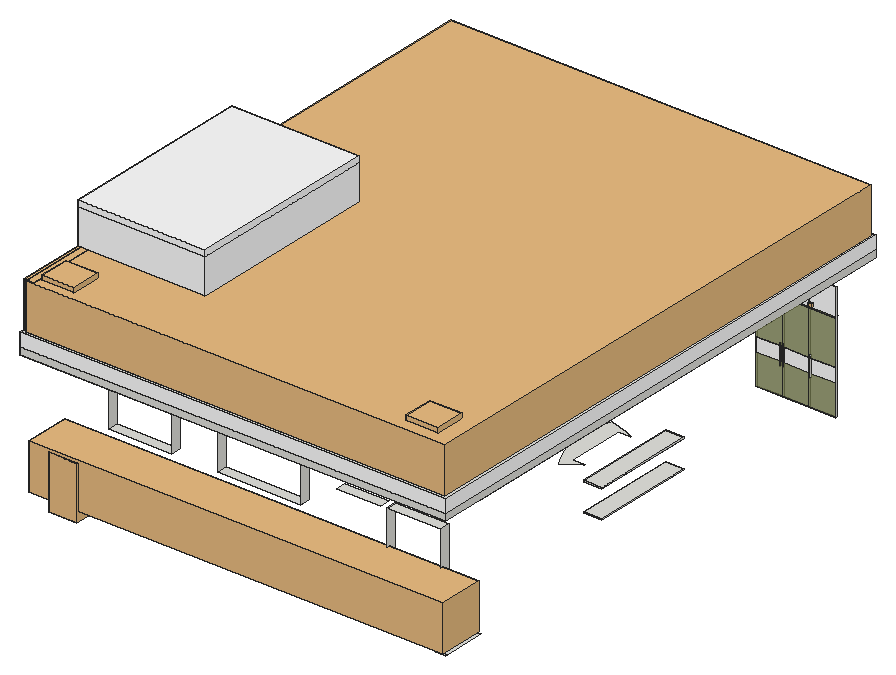
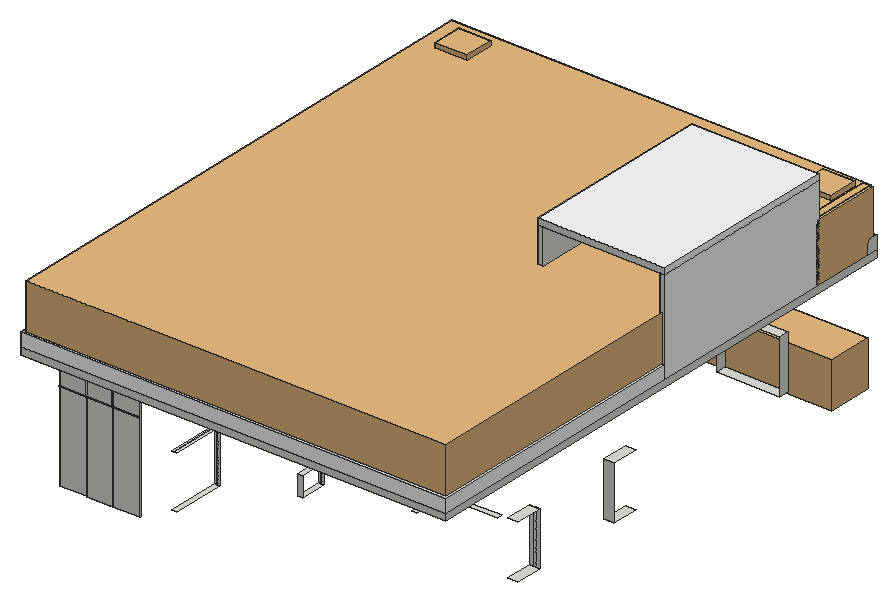
# SketchUp Ruby script. Lengths in inches.
U = 1.inch
M = Sketchup.active_model
def pt(a) = Geom::Point3d.new(a.map { |v| v * U })
def face(e, loops, mat)
  f = e.add_face(loops[0].map { |a| pt(a) })
  loops[1..].each { |l| e.add_face(l.map { |a| pt(a) }).erase! }
  f.material = f.back_material = mat if mat
  f
end
# faces: each face lists its corners as indices into pts; further lists are holes
def faces(e, pts, list, mat = nil) = list.each { |f| face(e, (f[0].is_a?(Array) ? f : [f]).map { |l| l.map { |i| pts[i] } }, mat) }
# xy, xz, yz: faces in a plane at the given z, y or x. An outline is a flat list of corners, or four numbers for a rectangle; further outlines are holes
def ring(l) = l.size == 4 ? [[l[0], l[1]], [l[2], l[1]], [l[2], l[3]], [l[0], l[3]]] : l.each_slice(2).to_a
def flat(e, list, mat, &to3) = list.each { |f| face(e, (f[0].is_a?(Array) ? f : [f]).map { |l| ring(l).map { |u, v| to3.(u, v) } }, mat) }
def xy(e, z, list, mat = nil) = flat(e, list, mat) { |x, y| [x, y, z] }
def xz(e, y, list, mat = nil) = flat(e, list, mat) { |x, z| [x, y, z] }
def yz(e, x, list, mat = nil) = flat(e, list, mat) { |y, z| [x, y, z] }
def lines(e, pts, list) = list.each { |a, b| e.add_line(pt(pts[a]), pt(pts[b])) }
# prism: a flat outline (further loops are holes) pulled along v
def prism(e, loops, v, mat = nil)
  f = face(e, loops, mat); d = Geom::Vector3d.new(v.map { |x| x * U })
  f.pushpull(f.normal.samedirection?(d) ? d.length : -d.length)
end
def box(e, o, s, mat = nil) = prism(e, [[o, [o[0] + s[0], o[1], o[2]], [o[0] + s[0], o[1] + s[1], o[2]], [o[0], o[1] + s[1], o[2]]]], [0, 0, s[2]], mat)
def at(x, y, z, deg = 0) = Geom::Transformation.translation(pt([x, y, z])) * Geom::Transformation.rotation(ORIGIN, Z_AXIS, deg.degrees)
def axes(o, x, y, z) = Geom::Transformation.new([*x, 0, *y, 0, *z, 0, *pt(o).to_a, 1])
def part(name) = M.definitions.add(name)
# library, detail: a bought-in or finely detailed component or shape, given as its bounding box
def library(name, o, s) = part(name).tap { |d| box(d.entities, o, s) }
def detail(e, o, s) = box(e.add_group.entities, o, s)
def put(e, d, t, mat = nil) = e.add_instance(d, t).tap { |i| i.material = mat if mat }
def group(e, t, mat = nil) = e.add_group.tap { |g| g.transformation = t; g.material = mat if mat }.entities
root = M.entities
M.materials.add("Acrylic Opaque Olive Green Rough 001").color = [133, 140, 86]
M.materials["Acrylic Opaque Olive Green Rough 001"].alpha = 0.73
M.materials.add("Acrylic Opaque Olive Green Rough 001\#1").color = [133, 140, 86]
M.materials["Acrylic Opaque Olive Green Rough 001\#1"].alpha = 0.73
M.materials.add("Ceramic Sand 8.13cm").color = [255, 255, 255]
M.materials.add("Manhattan Creative Coating MD 1125B 26.44cm").color = [255, 255, 255]
M.materials.add("Marble 001 38.37cm").color = [255, 255, 255]
c1 = library("Indoor Plant 010",[-15.15,-14.1,0],[25.78,27.29,47.64])
c2 = library("Group\#156",[0,0,0],[372.04,40.76,40.98])
c3 = part("OuterShell")
prism(c3.entities,[[[0,0,0.08],[0,0,0.31],[0,0.59,0.31],[0,0.59,0.39],[0,0.79,0.39],[0,0.79,0],[0,0.59,0],[0,0.59,0.08]]],[0.39,0,0])
c4 = part("Cabinet pull")
put(c4.entities,c3,at(0,0,0))
put(c4.entities,c3,at(8.62,0,0))
g1 = group(c4.entities,at(0,0,0))
g2 = group(g1,at(0,0,0.2))
xy(g2,0,[[0.39,0.39,8.62,0.79]])
xy(g2,0.12,[[0.39,0.39,8.62,0.59]])
xy(g2,0.2,[[0.39,0.59,8.62,0.63],[0.39,0.63,8.62,0.79]])
xz(g2,0.39,[[0.39,0,8.62,0.12]])
xz(g2,0.59,[[0.39,0.12,8.62,0.2]])
xz(g2,0.79,[[0.39,0,8.62,0.2]])
yz(g2,0.39,[[0.39,0,0.39,0.12,0.59,0.12,0.59,0.2,0.79,0.2,0.79,0]])
yz(g2,8.62,[[0.39,0,0.79,0,0.79,0.2,0.59,0.2,0.59,0.12,0.39,0.12]])
g3 = group(g1,at(0,0,0.2))
xy(g3,-0.2,[[0.39,0.59,8.62,0.63],[0.39,0.63,8.62,0.79]])
xy(g3,-0.12,[[0.39,0.39,8.62,0.59]])
xy(g3,0,[[0.39,0.39,8.62,0.79]])
xz(g3,0.39,[[0.39,-0.12,8.62,0]])
xz(g3,0.59,[[0.39,-0.2,8.62,-0.12]])
xz(g3,0.79,[[0.39,-0.2,8.62,0]])
yz(g3,0.39,[[0.59,-0.2,0.79,-0.2,0.79,0,0.39,0,0.39,-0.12,0.59,-0.12]])
yz(g3,8.62,[[0.59,-0.2,0.59,-0.12,0.39,-0.12,0.39,0,0.79,0,0.79,-0.2]])
c5 = part("Group\#64")
box(c5.entities,[0,0,0],[16.1875,92.01,1])
c6 = library("Sphere Light",[-2,-2,-2],[4,4,4])
c7 = part("door thingy")
detail(c7.entities,[0,0,0],[0.75,0.75,0.5])
c8 = part("Group1421\#1")
p = [[0,0,0],[0,0,-8.78],[-0.06,0,-8.78],[0.38,-28.03,0],[-0.38,-28.03,0],[0.38,28.03,0],
  [0.38,0,0],[-0.38,28.03,0],[0.06,0,-8.78],[-0.38,0,0],[0,0,-14.21]]
lines(c8.entities,p,[[0,1],[1,2],[3,4],[5,6],[7,5],[1,8],[9,0],[0,6],[8,10],[4,9],[6,3],[2,10],
  [9,7]])
c9 = part("Rectangle Light")
put(c9.entities,c8,at(0,0,0))
c10 = library("Tlon Light 650 Ceiling 152 007",[-12.8,-12.8,-3.78],[25.6,25.6,3.58])
c11 = library("Indoor Plant 004",[-26.75,-21.09,0],[44.44,41.03,87.36])
c12 = library("Group\#148",[0,0,0],[66.03,3.15,41.57])
c13 = library("Group\#150",[0,-4.9,0],[8.91,62.7,53.05])
c14 = library("Group\#152",[0,0,0],[376.52,477.15,40.98])
xy(root,264,[[409,155.96,413.5,194.96],[413.5,155.96,418,194.96]])
xy(root,288,[[334,194.96,382,203.96],[57.85,227.96,114,236.96],[156,227.96,230,236.96],[36,425.96,45,449.96],[36,533.96,45,557.96],
  [284.5,581.96,289,629.96]])
xy(root,296.25,[[344.58,374.48,359.39,384.71,348.58,384.71,348.58,436.62,359.39,436.62,359.39,436.68,352.48,439.22,335.58,445.43,333.68,439.54,332.25,433.51,331.31,427.39,330.86,421.22,330.9,415.03,331.43,408.86,332.46,402.75,333.96,396.75,335.94,390.88,338.38,385.19,341.27,379.71]])
xy(root,336,[[289,194.96,328,203.96],[334,194.96,382,203.96],[57.85,227.96,114,236.96],[236.5,227.96,275.5,236.96],[289,329.96,328,334.46],
  [171,421.46,210,425.96],[214.5,421.46,244.5,425.96],[36,425.96,45,449.96],[289,445.46,328,449.96],[284.5,527.96,289,557.96],
  [36,533.96,45,557.96],[51,557.96,87,562.46],[216,557.96,250,562.46],[99,562.46,103.5,592.46],[284.5,581.96,286.2,629.96],
  [286.2,581.96,287.3,629.96],[287.3,581.96,289,629.96],[175.5,601.46,180,625.46]])
xy(root,348,[[156,227.96,230,236.96]])
xy(root,354,[[216,557.96,250,562.46],[175.5,601.46,180,625.46]])
xy(root,372,[[[36,155.96,45,155.96,45,227.96,280,227.96,280,194.96,373,194.96,373,203.96,289,203.96,289,329.96,409,329.96,409,334.46,289,334.46,289,361.46,280,361.46,280,352.46,284.5,352.46,284.5,236.96,145.5,236.96,145.5,373.46,141,373.46,141,236.96,45,236.96,45,421.46,280,421.46,280,416.96,289,416.96,289,445.46,409,445.46,409,449.96,289,449.96,289,629.96,409,629.96,409,203.96,373,203.96,373,194.96,418,194.96,418,638.96,36,638.96],[45,425.96,45,629.96,99,629.96,99,562.46,45,562.46,45,557.96,210,557.96,210,425.96],[103.5,562.46,103.5,629.96,284.5,629.96,284.5,562.46,180,562.46,180,629.96,175.5,629.96,175.5,562.46],[214.5,425.96,214.5,557.96,284.5,557.96,284.5,467.96,214.5,467.96,214.5,463.46,284.5,463.46,284.5,425.96]]])
xy(root,462,[[36,220.77,150,392.96]])
xy(root,468,[[36,220.77,150,392.96]],"Ceramic Sand 8.13cm")
xz(root,220.77,[[36,462,150,468]],"Manhattan Creative Coating MD 1125B 26.44cm")
xz(root,392.96,[[36,462,150,468]])
xz(root,449.96,[[36,288,45,336]])
xz(root,533.96,[[36,288,39.7,336],[39.7,288,41.3,336],[41.3,288,45,336]])
xz(root,581.96,[[284.5,288,286.2,336],[286.2,288,287.3,336],[287.3,288,289,336]])
xz(root,601.46,[[175.5,336,177.2,354],[177.2,336,178.3,354],[178.3,336,180,354]])
xz(root,625.46,[[175.5,336,180,354]])
yz(root,36,[[220.77,462,392.96,468]],"Manhattan Creative Coating MD 1125B 26.44cm")
yz(root,57.85,[[227.96,288,236.96,336]])
yz(root,114,[[227.96,288,236.96,336]])
yz(root,150,[[220.77,462,392.96,468]],"Manhattan Creative Coating MD 1125B 26.44cm")
yz(root,156,[[227.96,288,236.96,348]])
yz(root,216,[[557.96,336,559.66,354],[559.66,336,560.76,354],[560.76,336,562.46,354]])
yz(root,230,[[227.96,288,236.96,348]])
yz(root,250,[[557.96,336,562.46,354]])
yz(root,334,[[194.96,288,203.96,336]])
yz(root,382,[[194.96,288,203.96,336]])
p = [[409,157.74,264],[418,157.74,264]]
lines(root,p,[[0,1]])
g4 = group(root,at(337,604.96,255))
xy(g4,0,[[0,0,23.97,1],[24.13,0,47.87,1],[48.03,0,72,1]])
xy(g4,79.69,[[23.97,0,24.13,1],[47.87,0,48.03,1]])
xy(g4,80.69,[[0.16,0,23.97,1.875],[23.97,0,24.13,1.875],[24.13,0,47.87,1.875],[47.87,0,48.03,1.875],[48.03,0,71.84,1.875]])
xy(g4,80.84,[[0.16,0,23.97,1.875],[24.13,0,47.87,1.875],[48.03,0,71.84,1.875],[23.97,1.875,24.13,1.9375]])
xy(g4,104.84,[[23.97,0,24.13,1.9375],[47.87,0,48.03,1.875]])
xy(g4,105,[[0,0,72,1]])
xz(g4,0,[[0.16,0,23.97,27.84],[24.13,0,47.87,27.84],[48.03,0,71.84,27.84],[0.16,39.84,23.97,79.69],[24.13,39.84,47.87,79.69],
  [48.03,39.84,71.84,79.69]],"Acrylic Opaque Olive Green Rough 001")
xz(g4,0,[[0,0,0.16,105],[71.84,0,72,105],[0.16,79.69,71.84,80.69],[0.16,104.84,71.84,105]],"Acrylic Opaque Olive Green Rough 001\#1")
xz(g4,0,[[0.16,27.84,23.97,39.84],[24.13,27.84,47.87,39.84],[48.03,27.84,71.84,39.84],[0.16,80.84,23.97,104.84],[24.13,80.84,47.87,104.84],
  [48.03,80.84,71.84,104.84]],"Marble 001 38.37cm")
xz(g4,1,[[0,0,0,105,72,105,72,0,48.03,0,48.03,79.69,47.87,79.69,47.87,0,24.13,0,24.13,79.69,23.97,79.69,23.97,0]])
xz(g4,1.875,[[0.16,80.69,71.84,80.84],[47.87,80.84,48.03,104.84]])
xz(g4,1.9375,[[23.97,80.84,24.13,104.84]])
yz(g4,0,[[0,0,1,105]])
yz(g4,0.16,[[0,80.69,1.875,80.84]])
yz(g4,23.97,[[0,0,1,79.69],[0,80.84,1.9375,104.84]])
yz(g4,24.13,[[0,0,1,79.69],[0,80.84,1.9375,104.84]])
yz(g4,47.87,[[0,0,1,79.69],[0,80.84,1.875,104.84]])
yz(g4,48.03,[[0,0,1,79.69],[0,80.84,1.875,104.84]])
yz(g4,71.84,[[0,80.69,1.875,80.84]])
yz(g4,72,[[0,0,1,105]])
p = [[47.87,0,39.84],[48.03,0,39.84],[23.97,0,39.84],[24.13,0,39.84],[47.87,0,27.84],[48.03,0,27.84],
  [23.97,0,27.84],[24.13,0,27.84]]
lines(g4,p,[[0,1],[2,3],[4,5],[6,7]])
put(root,c1,at(76.98,169.49,255.13))
put(root,c2,at(43.03,156.17,264))
put(root,c4,axes([359.55,604.96,279.69],[0,0,2.016],[0,-1,0],[1,0,0]))
put(root,c4,axes([386.05,604.96,279.69],[0,0,2.016],[0,-1,0],[1,0,0]))
put(root,c4,axes([362.05,604.96,279.69],[0,0,2.016],[0,-1,0],[1,0,0]))
put(root,c5,at(391,343.96,286.73))
put(root,c6,at(280.68,341.19,289.29))
put(root,c6,at(280.68,341.19,302.1875))
put(root,c5,at(391,343.96,311.96))
put(root,c6,at(280.68,341.19,315.23))
put(root,c6,at(280.68,341.19,328.23))
put(root,c7,axes([357.35,604.96,337.3],[3.9959,0,0],[0,0,3.9959],[0,-3.9959,0]))
put(root,c7,axes([361.72,604.96,337.3],[3.9959,0,0],[0,0,3.9959],[0,-3.9959,0]))
put(root,c7,axes([385.59,604.96,337.3],[3.9959,0,0],[0,0,3.9959],[0,-3.9959,0]))
put(root,c9,axes([282.12,307.81,343.22],[-1,0,0],[0,-1,0],[0,0,0.03614]))
put(root,c10,axes([78.61,183.63,372.11],[0.54,0,0],[0,0.54,0],[0,0,0.54]))
put(root,c10,axes([225.23,183.63,372.11],[0.54,0,0],[0,0.54,0],[0,0,0.54]))
put(root,c10,axes([366.98,183.63,372.11],[0.54,0,0],[0,0.54,0],[0,0,0.54]))
g5 = group(root,at(36,98.96,372))
prism(g5,[[[382,540,0],[382,57,0],[0,57,0],[0,540,0]],[[105,270,0],[9,270,0],[9,131,0],[105,131,0]]],[0,0,6])
put(root,c11,axes([388.53,183.52,378],[0.65,0,0],[0,0.65,0],[0,0,0.65]))
g6 = group(root,at(36,220.77,378))
xy(g6,0,[[0,0,0,172.1875,4.5,172.1875,4.5,4.5,109.5,4.5,109.5,172.1875,114,172.1875,114,0]])
xy(g6,84,[[0,0,114,0,114,172.1875,109.5,172.1875,109.5,4.5,4.5,4.5,4.5,172.1875,0,172.1875]])
xz(g6,0,[[0,0,114,84]],"Ceramic Sand 8.13cm")
xz(g6,4.5,[[4.5,0,109.5,84]])
xz(g6,172.1875,[[0,0,4.5,84],[109.5,0,114,84]])
yz(g6,0,[[0,0,172.1875,84]],"Ceramic Sand 8.13cm")
yz(g6,4.5,[[4.5,0,172.1875,84]])
yz(g6,109.5,[[4.5,0,172.1875,84]])
yz(g6,114,[[0,0,172.1875,84]],"Ceramic Sand 8.13cm")
put(root,c12,at(81.04,370.21,378))
g7 = group(root,at(36,155.96,378))
p = [[4.45,9.03,12.06],[4.45,0,12.0625]]
lines(g7,p,[[0,1]])
put(g7,c13,at(0,9,0))
g8 = group(g7,at(0,0,0))
xy(g8,0,[[0,0,0,9,373,9,373,473.99,9,473.99,9,237,0,237,0,483,382,483,382,0]])
xy(g8,12.0625,[[0,0,382,0,382,483,0,483,0,237,4.5,237,4.5,478.5,377.5,478.5,377.5,4.5,4.52,4.5,4.52,9,0,9],[4.52,4.5,377.5,4.5,377.5,478.5,4.5,478.5,4.5,237,9,237,9,473.99,373,473.99,373,9,4.52,9]])
xz(g8,0,[[0,0,382,12.0625]],"Manhattan Creative Coating MD 1125B 26.44cm")
xz(g8,9,[[0,0,373,12.0625]])
xz(g8,237,[[0,0,9,12.0625]])
xz(g8,473.99,[[9,0,373,12.0625]])
xz(g8,483,[[0,0,382,12.0625]],"Manhattan Creative Coating MD 1125B 26.44cm")
yz(g8,0,[[0,0,9,12.0625]])
yz(g8,0,[[237,0,483,12.0625]],"Manhattan Creative Coating MD 1125B 26.44cm")
yz(g8,9,[[237,0,473.99,12.0625]])
yz(g8,373,[[9,0,473.99,12.0625]])
yz(g8,382,[[0,0,483,12.0625]],"Manhattan Creative Coating MD 1125B 26.44cm")
put(g8,c14,at(2.55,2.93,12.0625))
put(root,c11,axes([63.98,180.85,378],[0.65,0,0],[0,0.65,0],[0,0,0.65]))
